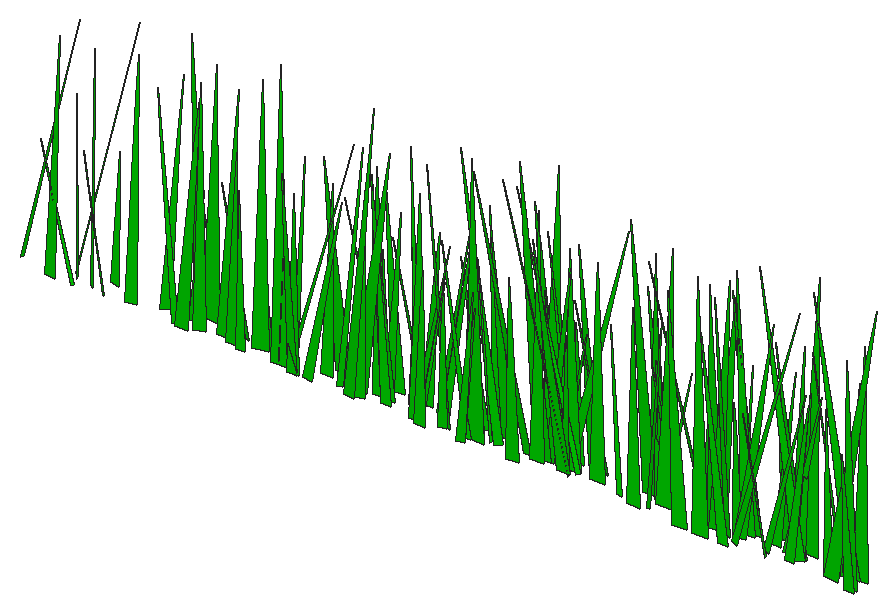
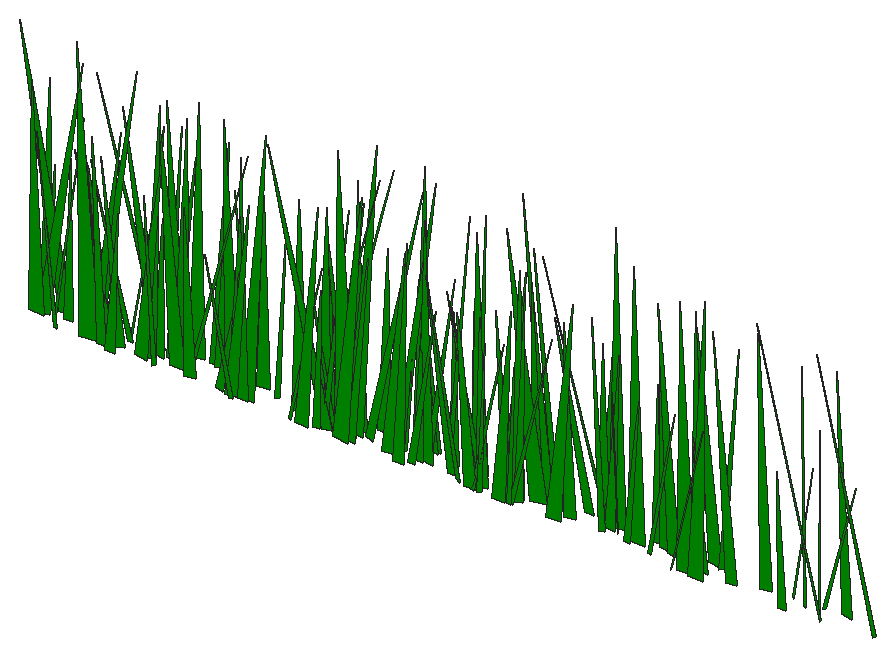
# SketchUp Ruby script. Lengths in inches.
U = 1.inch
M = Sketchup.active_model
def pt(a) = Geom::Point3d.new(a.map { |v| v * U })
def face(e, loops, mat)
  f = e.add_face(loops[0].map { |a| pt(a) })
  loops[1..].each { |l| e.add_face(l.map { |a| pt(a) }).erase! }
  f.material = f.back_material = mat if mat
  f
end
# faces: each face lists its corners as indices into pts; further lists are holes
def faces(e, pts, list, mat = nil) = list.each { |f| face(e, (f[0].is_a?(Array) ? f : [f]).map { |l| l.map { |i| pts[i] } }, mat) }
# xy, xz, yz: faces in a plane at the given z, y or x. An outline is a flat list of corners, or four numbers for a rectangle; further outlines are holes
def ring(l) = l.size == 4 ? [[l[0], l[1]], [l[2], l[1]], [l[2], l[3]], [l[0], l[3]]] : l.each_slice(2).to_a
def flat(e, list, mat, &to3) = list.each { |f| face(e, (f[0].is_a?(Array) ? f : [f]).map { |l| ring(l).map { |u, v| to3.(u, v) } }, mat) }
def xy(e, z, list, mat = nil) = flat(e, list, mat) { |x, y| [x, y, z] }
def xz(e, y, list, mat = nil) = flat(e, list, mat) { |x, z| [x, y, z] }
def yz(e, x, list, mat = nil) = flat(e, list, mat) { |y, z| [x, y, z] }
def lines(e, pts, list) = list.each { |a, b| e.add_line(pt(pts[a]), pt(pts[b])) }
# prism: a flat outline (further loops are holes) pulled along v
def prism(e, loops, v, mat = nil)
  f = face(e, loops, mat); d = Geom::Vector3d.new(v.map { |x| x * U })
  f.pushpull(f.normal.samedirection?(d) ? d.length : -d.length)
end
def box(e, o, s, mat = nil) = prism(e, [[o, [o[0] + s[0], o[1], o[2]], [o[0] + s[0], o[1] + s[1], o[2]], [o[0], o[1] + s[1], o[2]]]], [0, 0, s[2]], mat)
def at(x, y, z, deg = 0) = Geom::Transformation.translation(pt([x, y, z])) * Geom::Transformation.rotation(ORIGIN, Z_AXIS, deg.degrees)
def axes(o, x, y, z) = Geom::Transformation.new([*x, 0, *y, 0, *z, 0, *pt(o).to_a, 1])
def part(name) = M.definitions.add(name)
# library, detail: a bought-in or finely detailed component or shape, given as its bounding box
def library(name, o, s) = part(name).tap { |d| box(d.entities, o, s) }
def detail(e, o, s) = box(e.add_group.entities, o, s)
def put(e, d, t, mat = nil) = e.add_instance(d, t).tap { |i| i.material = mat if mat }
def group(e, t, mat = nil) = e.add_group.tap { |g| g.transformation = t; g.material = mat if mat }.entities
root = M.entities
M.materials.add("[Color G06]").color = [0, 204, 0]
c1 = part("fur_instance\#9")
p = [[0.8125,0,1.79],[0.67,-0.02,1.48],[0,-0.11,0],[0,0.11,0]]
faces(c1.entities,p,[[0,1,2,3]])
put(root,c1,axes([95.6,20.95,4.28],[0.10173,-0.50966,1.57038],[-3.80172,-0.01737,-0.09756],[-0.09712,0.14617,5.4638]),"[Color G06]")
put(root,c1,axes([89.42,20.86,4.28],[-0.62404,0.40067,1.88586],[3.11451,0.10105,-0.16401],[0.38431,-0.16829,4.39138]),"[Color G06]")
put(root,c1,axes([108.33,20.83,4.28],[-2.65762,0.59389,2.57331],[4.4676,0.39872,-0.26433],[1.06955,-0.18976,7.49832]),"[Color G06]")
put(root,c1,axes([109.89,20.81,4.28],[-3.25741,0.37792,1.00856],[2.73299,0.4611,-0.13121],[0.57549,-0.05064,6.33179]),"[Color G06]")
put(root,c1,axes([118.23,21.03,4.28],[-0.44079,-0.39642,0.68795],[-2.87959,0.06156,-0.04659],[0.03932,0.0641,4.29934]),"[Color G06]")
put(root,c1,axes([106.95,20.84,4.28],[-2.15271,0.57883,1.69248],[4.27827,0.30673,0.10443],[0.45746,-0.14478,6.98779]),"[Color G06]")
put(root,c1,axes([80.71,21.04,4.28],[2.47498,0.33092,3.40143],[2.94863,-0.39915,-0.33161],[-1.45496,-0.24599,5.11401]),"[Color G06]")
put(root,c1,axes([92.1875,20.84,4.28],[1.692,0.3784,0.67249],[2.71823,-0.2413,0.31993],[-0.42097,-0.03717,4.76873]),"[Color G06]")
put(root,c1,axes([106.74,20.93,4.28],[-2.05883,0.32303,1.42525],[2.41631,0.3015,-0.05317],[0.66127,-0.09594,4.63172]),"[Color G06]")
put(root,c1,axes([88.95,21.22,4.28],[1.19381,-0.68945,0.62071],[-4.95762,-0.16815,-0.157],[-0.19991,0.05283,7.60025]),"[Color G06]")
put(root,c1,axes([89.36,21.06,4.28],[3.06955,-0.13381,0.6777],[-0.95776,-0.43261,-0.12259],[-0.45736,0.00784,4.80507]),"[Color G06]")
put(root,c1,axes([92.17,20.97,4.28],[1.94479,0.28009,0.88914],[2.045,-0.27839,0.08259],[-0.45433,-0.05411,4.17777]),"[Color G06]")
put(root,c1,axes([84.57,20.95,4.28],[4.79927,0.49224,2.33199],[3.63213,-0.69345,0.11758],[-1.305,-0.11977,8.9034]),"[Color G06]")
put(root,c1,axes([80.75,21,4.28],[0.69913,0.50661,1.05062],[3.68048,-0.10553,0.37495],[-0.3833,-0.08931,5.51669]),"[Color G06]")
put(root,c1,axes([85.1,21.2,4.28],[3.11001,-0.35699,2.30096],[-2.74142,-0.46419,0.0038],[-1.1869,0.13673,6.02039]),"[Color G06]")
put(root,c1,axes([81.72,21.04,4.28],[2.7915,0.41826,0.34946],[3.0066,-0.38943,-0.10401],[-0.10825,-0.03049,6.12307]),"[Color G06]")
put(root,c1,axes([112.46,21.2,4.28],[-2.8299,0.00335,0.68701],[0.04467,0.39937,0.18733],[0.45812,-0.01825,4.22549]),"[Color G06]")
put(root,c1,axes([64.25,21.1875,4.28],[-3.04216,-0.43021,3.77831],[-3.61669,0.48448,-0.16768],[1.6819,0.26365,6.4735]),"[Color G06]")
put(root,c1,axes([92.73,21.375,4.28],[-1.12099,-0.77001,2.54817],[-5.75658,0.17017,0.25028],[0.51051,0.22804,8.41759]),"[Color G06]")
put(root,c1,axes([65.73,21.25,4.28],[-2.89994,0.07736,0.14424],[0.55579,0.40457,0.03564],[0.09031,-0.0058,4.41262]),"[Color G06]")
put(root,c1,axes([77.04,21.25,4.28],[-1.97424,0.3268,1.73195],[2.48127,0.298,-0.14153],[0.82367,-0.11443,4.57762]),"[Color G06]")
put(root,c1,axes([103.61,21.18,4.28],[-1.34823,0.52339,1.37649],[3.83473,0.19808,-0.26188],[0.48029,-0.11227,5.95483]),"[Color G06]")
put(root,c1,axes([90.54,21.38,4.28],[1.47188,-0.37292,1.16283],[-2.72628,-0.21801,-0.32319],[-0.56971,0.07981,4.55085]),"[Color G06]")
put(root,c1,axes([118.1,21.32,4.28],[-1.99109,-0.53085,2.7512],[-4.15482,0.29836,-0.10334],[0.78637,0.23229,6.42007]),"[Color G06]")
put(root,c1,axes([79.61,21.33,4.28],[3.49987,-0.61109,3.88421],[-4.84799,-0.53465,0.09496],[-1.567,0.28925,8.38154]),"[Color G06]")
put(root,c1,axes([73.12,21.19,4.28],[2.52831,0.58351,1.22922],[4.21918,-0.36166,0.33679],[-0.62045,-0.08158,7.29921]),"[Color G06]")
put(root,c1,axes([92.3,21.3125,4.28],[-3.61982,0.21223,0.93655],[1.52692,0.51182,-0.14069],[0.61443,-0.0216,5.86714]),"[Color G06]")
put(root,c1,axes([67.7,21.38,4.28],[-2.769,-0.08918,0.84502],[-0.68287,0.392,-0.24599],[0.5122,0.04051,4.24029]),"[Color G06]")
put(root,c1,axes([110.29,21.31,4.28],[5.30648,0.27793,0.15561],[1.99562,-0.73946,-0.29666],[-0.0276,-0.03102,8.4667]),"[Color G06]")
put(root,c1,axes([72.54,21.35,4.28],[-4.37816,0.18589,1.91389],[1.32373,0.63573,-0.32891],[1.29018,-0.02147,6.83216]),"[Color G06]")
put(root,c1,axes([104.41,21.41,4.28],[3.5971,0.15603,1.71417],[1.09089,-0.52636,0.39052],[-1.17366,-0.01102,5.61668]),"[Color G06]")
put(root,c1,axes([83.54,21.49,4.28],[4.87808,-0.13743,2.05158],[-1.04859,-0.70475,0.14635],[-1.32512,0.05178,7.43651]),"[Color G06]")
put(root,c1,axes([98.46,21.68,4.28],[-2.5032,-0.58164,0.68581],[-4.19377,0.34931,-0.16044],[0.14361,0.06259,7.26865]),"[Color G06]")
put(root,c1,axes([74.03,21.56,4.28],[3.51268,-0.45111,2.82056],[-3.42534,-0.53287,-0.2614],[-1.51465,0.15887,7.1324]),"[Color G06]")
put(root,c1,axes([98.8,21.6,4.28],[-5.90337,-0.14529,0.45081],[-1.0299,0.82382,0.37449],[0.34039,-0.02715,8.95156]),"[Color G06]")
put(root,c1,axes([84.54,21.79,4.28],[2.77635,-0.703,0.04507],[-5.03842,-0.38674,0.32308],[0.17482,0.01822,8.59565]),"[Color G06]")
put(root,c1,axes([80.2,21.41,4.28],[5.31263,0.21921,0.01045],[1.57086,-0.74039,0.28572],[-0.06094,0.02529,8.27551]),"[Color G06]")
put(root,c1,axes([86.64,21.48,4.28],[-1.70442,0.40952,1.01512],[2.99413,0.24257,-0.01165],[0.34781,-0.08136,5.07484]),"[Color G06]")
put(root,c1,axes([69.36,21.6,4.28],[-3.48196,0.41679,3.64932],[3.35929,0.55306,-0.09646],[1.90017,-0.21401,6.8577]),"[Color G06]")
put(root,c1,axes([90.73,21.63,4.28],[-4.74591,-0.26472,2.18451],[-1.94862,0.68962,0.14355],[1.39395,0.06275,7.63818]),"[Color G06]")
put(root,c1,axes([79.83,21.68,4.28],[-1.41523,-0.45189,1.43248],[-3.36095,0.20332,-0.049],[0.35244,0.12437,5.28483]),"[Color G06]")
put(root,c1,axes([102.32,21.56,4.28],[-3.09227,0.16479,1.49158],[1.15538,0.45291,-0.39758],[1.02841,-0.01333,4.93162]),"[Color G06]")
put(root,c1,axes([76.18,21.55,4.28],[1.49296,0.5011,1.35278],[3.66454,-0.21988,0.32244],[-0.55128,-0.10453,5.80693]),"[Color G06]")
put(root,c1,axes([88.69,21.64,4.28],[4.76425,-0.12245,3.7662],[-1.05654,-0.74686,0.19603],[-2.45047,0.08394,7.2378]),"[Color G06]")
put(root,c1,axes([116.68,21.47,4.28],[3.97247,0.64513,0.78581],[4.64772,-0.55521,-0.12163],[-0.28051,-0.06304,9.1129]),"[Color G06]")
put(root,c1,axes([113.77,21.56,4.28],[1.80615,0.41596,0.48317],[2.99344,-0.2534,0.06499],[-0.20479,-0.03541,5.21141]),"[Color G06]")
put(root,c1,axes([96.68,21.69,4.28],[-3.12285,0.49854,3.04278],[3.83942,0.48121,-0.25509],[1.47832,-0.19664,7.09015]),"[Color G06]")
put(root,c1,axes([109.44,21.78,4.28],[-4.04941,-0.31102,2.22835],[-2.27138,0.59778,0.36462],[1.42781,0.06886,6.89986]),"[Color G06]")
put(root,c1,axes([66.64,21.74,4.28],[-4.26697,-0.16867,3.13472],[-1.31792,0.65895,0.06583],[2.03108,0.07323,6.62827]),"[Color G06]")
put(root,c1,axes([110.17,21.92,4.28],[3.68569,-0.48522,0.47887],[-3.48653,-0.51499,-0.0028],[-0.23427,0.03048,7.57564]),"[Color G06]")
put(root,c1,axes([86.42,21.91,4.28],[-1.50408,-0.61789,1.15162],[-4.49309,0.21146,-0.07478],[0.19964,0.10401,6.99322]),"[Color G06]")
put(root,c1,axes([98.53,21.76,4.28],[-1.6103,-0.27853,1.72],[-2.17324,0.24871,0.08163],[0.76874,0.11967,3.8337]),"[Color G06]")
put(root,c1,axes([79.22,21.79,4.28],[2.67603,0.01852,1.48896],[0.23283,-0.39579,-0.36905],[-0.97772,-0.04355,3.9874]),"[Color G06]")
put(root,c1,axes([93.48,21.79,4.28],[-3.48623,0.03909,1.61797],[0.29292,0.5089,-0.00253],[1.07922,-0.01185,5.22724]),"[Color G06]")
put(root,c1,axes([108.6,21.86,4.28],[3.64882,-0.49287,2.30196],[-3.70244,-0.53042,0.063],[-1.0756,0.15384,7.5922]),"[Color G06]")
put(root,c1,axes([112.13,21.72,4.28],[3.15318,0.28404,0.20229],[2.04139,-0.43897,-0.27263],[-0.01451,-0.03161,5.60384]),"[Color G06]")
put(root,c1,axes([108.52,21.97,4.28],[-1.2927,-0.67785,1.62422],[-4.9569,0.19046,0.31862],[0.48982,0.1385,7.51094]),"[Color G06]")
put(root,c1,axes([109.97,21.96,4.28],[0.31948,-0.406,0.47592],[-2.92532,-0.04644,-0.16462],[-0.14484,0.04242,4.37453]),"[Color G06]")
put(root,c1,axes([88.48,21.75,4.28],[3.25566,0.29387,0.42718],[2.10653,-0.45562,0.14427],[-0.29246,-0.01032,5.7945]),"[Color G06]")
put(root,c1,axes([96.77,22.02,4.28],[-2.32371,-0.77364,2.00417],[-5.69663,0.32692,-0.25702],[0.35532,0.1819,8.98607]),"[Color G06]")
put(root,c1,axes([95.8,21.97,4.28],[-5.03274,-0.37993,0.82377],[-2.75644,0.70264,-0.38927],[0.35963,0.06864,8.54448]),"[Color G06]")
put(root,c1,axes([77.79,21.98,4.28],[2.61871,-0.6627,2.48975],[-4.93854,-0.38919,-0.29713],[-0.98556,0.18932,8.10433]),"[Color G06]")
put(root,c1,axes([116.14,21.93,4.28],[-2.16623,0.29077,2.1881],[2.38222,0.32618,0.28888],[0.9035,-0.16288,4.4845]),"[Color G06]")
put(root,c1,axes([93.95,21.86,4.28],[-5.38066,0.30884,1.73044],[2.30257,0.76162,0.37803],[0.97149,-0.09465,8.68816]),"[Color G06]")
put(root,c1,axes([65.46,21.98,4.28],[-3.45748,-0.03553,2.31863],[-0.16157,0.52789,0.39096],[1.56382,-0.024,5.1667]),"[Color G06]")
put(root,c1,axes([61.73,21.97,4.28],[5.67279,-0.04551,0.56992],[-0.32778,-0.79282,0.01593],[-0.38009,0.00454,8.4924]),"[Color G06]")
put(root,c1,axes([75.38,21.86,4.28],[3.26583,0.53992,1.90722],[3.9562,-0.47477,0.30755],[-0.98429,-0.11683,7.56426]),"[Color G06]")
put(root,c1,axes([85.83,22.02,4.28],[0.30911,0.59463,2.8383],[4.66019,-0.05466,0.18167],[-0.26991,-0.26268,6.38736]),"[Color G06]")
put(root,c1,axes([114.13,21.96,4.28],[-5.11722,0.38251,1.51125],[2.82025,0.72076,0.37458],[0.77017,-0.09782,8.66951]),"[Color G06]")
put(root,c1,axes([99.24,22.01,4.28],[-5.73644,0.12096,0.45779],[0.88076,0.80004,0.36841],[0.26568,-0.04041,8.66318]),"[Color G06]")
put(root,c1,axes([104.9,22.1,4.28],[2.42569,-0.63091,2.58997],[-4.79247,-0.35212,0.17266],[-0.71115,0.22095,7.67069]),"[Color G06]")
put(root,c1,axes([113.18,22.1875,4.28],[2.91197,-0.35953,0.03438],[-2.57696,-0.40566,0.23217],[0.08577,0.01834,5.8083]),"[Color G06]")
put(root,c1,axes([82.26,22.03,4.28],[1.75847,-0.43965,2.53628],[-3.52973,-0.2571,0.34701],[-0.60084,0.22366,5.38431]),"[Color G06]")
put(root,c1,axes([80.03,22.07,4.28],[3.81426,-0.19261,2.17656],[-1.4949,-0.56361,0.12227],[-1.33941,0.08053,6.06174]),"[Color G06]")
put(root,c1,axes([114.11,22.16,4.28],[2.70048,-0.31303,1.20998],[-2.25909,-0.39027,-0.33599],[-0.76877,0.04728,5.23765]),"[Color G06]")
put(root,c1,axes([78.28,22.15,4.28],[-2.13424,-0.27327,1.1405],[-2.02384,0.3081,0.02065],[0.57174,0.0705,4.33047]),"[Color G06]")
put(root,c1,axes([90.05,22.21,4.28],[3.75287,-0.29493,0.77795],[-2.11005,-0.52814,-0.26401],[-0.54044,0.01399,6.43296]),"[Color G06]")
put(root,c1,axes([91.96,22.06,4.28],[0.72127,0.65633,2.3581],[4.95008,-0.11179,0.19228],[-0.37287,-0.21453,7.11402]),"[Color G06]")
put(root,c1,axes([100.49,22,4.28],[-0.9564,0.60852,1.28998],[4.437,0.13929,-0.20014],[0.31792,-0.11344,6.67388]),"[Color G06]")
put(root,c1,axes([97.18,22.07,4.28],[2.80168,0.42159,1.27001],[3.0966,-0.39731,-0.10839],[-0.52318,-0.09392,6.15952]),"[Color G06]")
put(root,c1,axes([114.04,22.32,4.28],[-2.7403,-0.49932,0.69625],[-3.58933,0.38557,0.20833],[0.39426,0.03969,6.73579]),"[Color G06]")
put(root,c1,axes([92.32,22.24,4.28],[0.11671,-0.37591,0.98387],[-2.77225,-0.01987,-0.13757],[-0.12312,0.09109,4.03045]),"[Color G06]")
put(root,c1,axes([116.86,22.15,4.28],[-4.36114,0.01641,1.28463],[0.09271,0.61962,-0.2064],[0.86258,0.01639,6.51715]),"[Color G06]")
put(root,c1,axes([98.83,22.05,4.28],[-1.11542,0.60445,1.50871],[4.4434,0.15953,-0.00421],[0.25436,-0.13622,6.68955]),"[Color G06]")
put(root,c1,axes([71.15,22.28,4.28],[4.22099,-0.36259,1.7808],[-2.62199,-0.60887,-0.35915],[-1.1429,0.0577,7.40084]),"[Color G06]")
put(root,c1,axes([87.93,22.35,4.28],[0.13256,-0.48674,0.86213],[-3.53597,-0.01558,0.20389],[0.11629,0.08105,5.21664]),"[Color G06]")
put(root,c1,axes([73.06,22.16,4.28],[1.67368,0.31072,0.66008],[2.23411,-0.239,0.27037],[-0.41113,-0.0338,4.15634]),"[Color G06]")
put(root,c1,axes([107.58,22.34,4.28],[-5.09039,-0.19196,0.28244],[-1.37526,0.71032,0.0918],[0.19846,-0.00139,7.88072]),"[Color G06]")
put(root,c1,axes([98,22.21,4.28],[2.56918,0.21214,0.41357],[1.50867,-0.36031,0.29603],[-0.33893,0.00425,4.45269]),"[Color G06]")
put(root,c1,axes([97.58,22.26,4.28],[-2.54406,0.30783,1.22596],[2.26525,0.36591,-0.05414],[0.64395,-0.07103,5.03388]),"[Color G06]")
put(root,c1,axes([117.63,22.1875,4.28],[-4.66835,0.46848,1.00313],[3.38834,0.65474,0.09739],[0.50642,-0.06209,8.59556]),"[Color G06]")
put(root,c1,axes([94.1,22.52,4.28],[-1.67463,-0.56406,0.50298],[-4.04747,0.23588,0.28532],[0.30551,0.03311,6.53694]),"[Color G06]")
put(root,c1,axes([76.57,22.41,4.28],[-2.89991,-0.17358,0.60912],[-1.24038,0.40829,0.17492],[0.4208,0.00728,4.71331]),"[Color G06]")
put(root,c1,axes([98.47,22.42,4.28],[-4.48748,0.11112,1.73387],[0.86412,0.64422,0.25264],[1.11095,-0.05222,6.80711]),"[Color G06]")
put(root,c1,axes([112.19,22.47,4.28],[2.69534,-0.35573,1.31576],[-2.65941,-0.3796,0.37949],[-0.45851,0.11062,5.53357]),"[Color G06]")
put(root,c1,axes([118.02,22.3,4.28],[1.06799,0.6417,1.81106],[4.73795,-0.15953,0.25204],[-0.44336,-0.15901,7.056]),"[Color G06]")
put(root,c1,axes([82.82,22.69,4.28],[-1.43507,-0.6477,0.03706],[-4.64177,0.20011,0.25653],[0.17131,-0.00376,7.26134]),"[Color G06]")
put(root,c1,axes([98.17,22.59,4.28],[5.23757,-0.35536,0.03056],[-2.54834,-0.73036,-0.01836],[-0.02376,-0.00029,8.70532]),"[Color G06]")
put(root,c1,axes([85.41,22.39,4.28],[-3.3788,0.34392,2.02279],[2.52166,0.50101,-0.3765],[1.24729,-0.08125,6.24073]),"[Color G06]")
put(root,c1,axes([65.01,22.47,4.28],[5.9876,0.06257,0.54405],[0.45544,-0.8363,-0.14761],[-0.35556,-0.01755,8.97279]),"[Color G06]")
put(root,c1,axes([108.45,22.33,4.28],[1.2976,0.66867,1.15211],[4.85602,-0.18062,-0.17463],[-0.08716,-0.10804,7.42254]),"[Color G06]")
put(root,c1,axes([110.3,22.45,4.28],[3.20641,-0.45281,4.18817],[-3.82466,-0.52267,0.04908],[-1.94144,0.28182,6.82034]),"[Color G06]")
put(root,c1,axes([114.05,22.79,4.28],[1.26381,-0.82732,1.33959],[-5.99993,-0.17287,0.37938],[0.06439,0.12959,9.05824]),"[Color G06]")
put(root,c1,axes([103.51,22.65,4.28],[-3.2604,-0.59376,2.32681],[-4.4547,0.46925,-0.18759],[0.84246,0.1834,8.01303]),"[Color G06]")
put(root,c1,axes([107.3125,22.73,4.28],[0.74601,-0.47861,0.59718],[-3.45537,-0.103,0.15876],[0.01964,0.05759,5.24712]),"[Color G06]")
put(root,c1,axes([110.625,22.68,4.28],[-2.77282,-0.5543,1.74151],[-4.11401,0.39132,-0.32364],[0.48331,0.1509,7.23635]),"[Color G06]")
put(root,c1,axes([73.79,22.83,4.28],[0.49178,-0.78164,1.06911],[-5.64776,-0.06469,0.36985],[0.18604,0.10231,8.40168]),"[Color G06]")
put(root,c1,axes([89.375,22.54,4.28],[3.72404,0.26043,0.78414],[1.85095,-0.52443,0.37193],[-0.58059,-0.00147,6.21541]),"[Color G06]")
put(root,c1,axes([105.3,22.75,4.28],[-1.72243,-0.32666,0.26362],[-2.34702,0.23796,-0.38087],[-0.1016,0.04083,4.32899]),"[Color G06]")
put(root,c1,axes([85.83,22.73,4.28],[2.65949,-0.37121,1.34378],[-2.72956,-0.38228,-0.06411],[-0.66662,0.08434,5.62355]),"[Color G06]")
put(root,c1,axes([104.3125,22.6,4.28],[0.45059,0.41882,1.33232],[3.11517,-0.07327,0.2926],[-0.33375,-0.11845,4.52975]),"[Color G06]")
put(root,c1,axes([67.41,22.71,4.28],[-1.05383,-0.3238,1.66245],[-2.48241,0.17226,0.33922],[0.68335,0.12641,3.79607]),"[Color G06]")
put(root,c1,axes([85.625,22.8,4.28],[-3.61003,-0.22786,0.15858],[-1.62875,0.50336,0.26208],[0.1689,-0.01619,5.91664]),"[Color G06]")
put(root,c1,axes([97.02,22.46,4.28],[-0.22468,0.86413,1.01324],[6.2323,0.03329,-0.17415],[0.1417,-0.09387,9.26623]),"[Color G06]")
put(root,c1,axes([92.41,22.68,4.28],[-2.86617,0.26147,0.82228],[1.92502,0.40121,0.33259],[0.33604,-0.06821,5.10815]),"[Color G06]")
put(root,c1,axes([96.38,22.81,4.28],[-2.62042,-0.39097,1.31965],[-2.87276,0.37556,0.03961],[0.62276,0.08736,5.73552]),"[Color G06]")
put(root,c1,axes([104.44,22.52,4.28],[-0.55403,0.56855,0.08494],[4.07478,0.0769,0.24105],[-0.15218,-0.01088,6.14499]),"[Color G06]")
put(root,c1,axes([88.18,22.84,4.28],[-3.09248,-0.19459,0.39091],[-1.3893,0.43277,0.19708],[0.29262,-0.00182,5.06689]),"[Color G06]")
put(root,c1,axes([85.71,22.86,4.28],[-2.50979,0.10685,1.61983],[0.92107,0.37297,0.36162],[0.95572,-0.07885,3.90528]),"[Color G06]")
put(root,c1,axes([103.72,22.85,4.28],[2.60471,0.50935,3.10751],[4.04485,-0.39646,-0.1083],[-1.142,-0.2425,6.70415]),"[Color G06]")
put(root,c1,axes([87.73,22.82,4.28],[-2.69123,0.17305,1.51222],[1.26106,0.39911,-0.23341],[0.98665,-0.0381,4.4231]),"[Color G06]")
put(root,c1,axes([96.92,23,4.28],[-1.96401,-0.65856,1.54632],[-4.82908,0.27475,-0.25879],[0.23393,0.1426,7.64013]),"[Color G06]")
put(root,c1,axes([98.7,22.84,4.28],[1.80533,-0.24436,2.1381],[-2.02057,-0.28895,0.0175],[-1.01713,0.14029,3.7602]),"[Color G06]")
put(root,c1,axes([100.42,22.9375,4.28],[-3.36468,-0.13759,0.4914],[-0.98316,0.47142,0.12597],[0.33924,0.00157,5.23902]),"[Color G06]")
put(root,c1,axes([109.61,22.88,4.28],[3.15253,-0.10053,1.70564],[-0.83963,-0.4626,0.33453],[-1.05693,0.06766,4.82172]),"[Color G06]")
put(root,c1,axes([99.51,23.06,4.28],[-1.90395,-0.58528,1.23263],[-4.26177,0.27034,0.04143],[0.36634,0.10311,6.88819]),"[Color G06]")
put(root,c1,axes([73,23.03,4.28],[-2.79973,-0.66877,2.45721],[-4.97257,0.41329,0.26584],[0.98865,0.18485,8.29558]),"[Color G06]")
put(root,c1,axes([113.11,22.92,4.28],[2.52073,0.42671,2.21743],[3.30695,-0.36763,-0.27047],[-0.7932,-0.17665,5.91918]),"[Color G06]")
put(root,c1,axes([88.36,22.8,4.28],[0.66606,0.51009,0.70842],[3.68823,-0.0912,-0.20258],[0.04958,-0.0684,5.55332]),"[Color G06]")
put(root,c1,axes([116.19,22.98,4.28],[3.57938,0.17779,1.55938],[1.34904,-0.51604,-0.15808],[-0.94568,-0.06321,5.6767]),"[Color G06]")
put(root,c1,axes([93.01,23,4.28],[-3.14118,0.39878,2.51858],[3.12146,0.46492,0.23987],[1.12896,-0.17589,6.34439]),"[Color G06]")
put(root,c1,axes([74.66,22.99,4.28],[-3.29913,-0.00496,0.38782],[-0.05309,0.46039,-0.33236],[0.25647,0.03149,4.91987]),"[Color G06]")
put(root,c1,axes([104.42,22.86,4.28],[-2.51378,0.49537,0.58647],[3.55971,0.353,-0.16978],[0.31969,-0.03546,6.50198]),"[Color G06]")
put(root,c1,axes([86.37,22.89,4.28],[-1.73316,0.53547,0.80475],[3.87273,0.24315,0.04507],[0.19379,-0.07018,6.2965]),"[Color G06]")
put(root,c1,axes([112.3,23.21,4.28],[-0.65008,-0.41613,0.1263],[-2.98202,0.09108,0.18915],[0.14168,0.00775,4.56077]),"[Color G06]")
put(root,c1,axes([104.23,23.125,4.28],[2.7257,-0.12838,0.36016],[-0.92417,-0.3814,0.00534],[-0.22716,0.01123,4.29987]),"[Color G06]")
